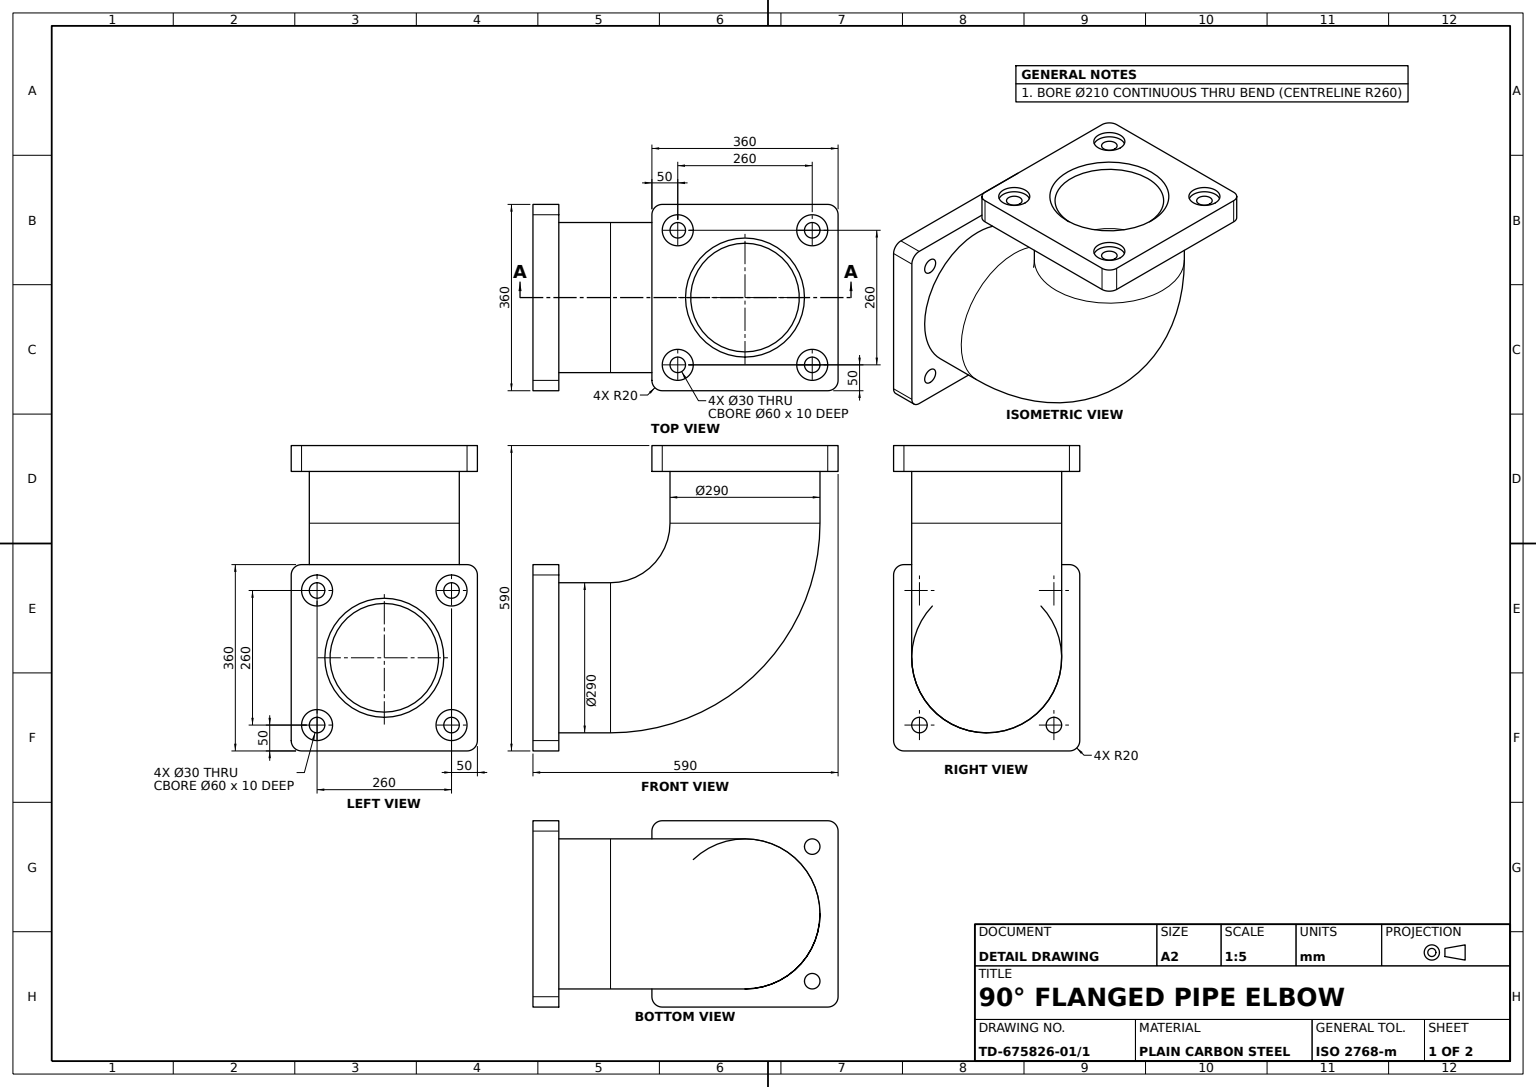
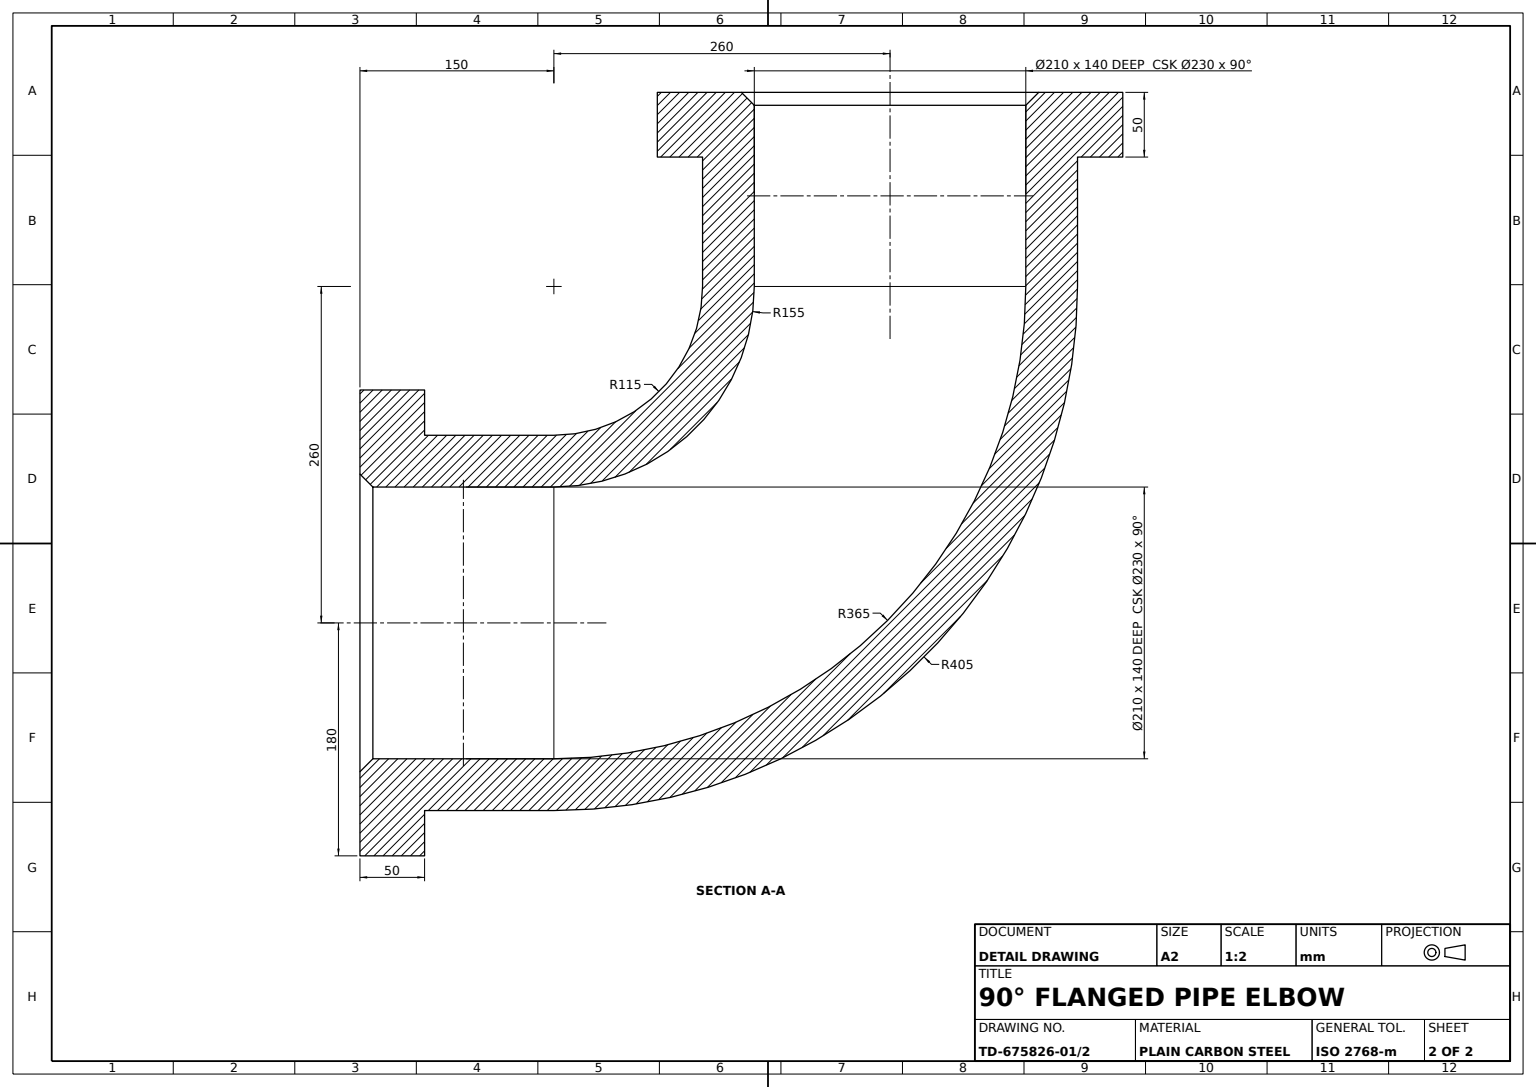
solid
v1 (0,260,-145)
v2 (-145,260,0)
e1 v1 v2 CIRCLE(AX(P(0,260,0),D(0,1,0),D(-1,0,0)),145)
v3 (0,260,145)
e2 v2 v3 CIRCLE(AX(P(0,260,0),D(0,1,0),D(-1,0,0)),145)
v4 (0,360,145)
e3 v4 v3 LINE
v5 (0,360,-145)
e4 v5 v4 CIRCLE(AX(P(0,360,0),D(0,1,0),D(-1,0,0)),145)
e5 v5 v1 LINE
face CYL(AX(P(0,410,0),D(0,-1,0),D(0,0,-1)),145) [e1 e2 -e3 -e4 e5]
v6 (-360,160,-180)
v7 (-410,160,-180)
e6 v6 v7 LINE
v8 (-360,-160,-180)
e7 v6 v8 LINE
v9 (-410,-160,-180)
e8 v8 v9 LINE
e9 v7 v9 LINE
face PLANE(AX(P(-360,160,-180),D(0,0,-1),D(0,1,0))) [-e6 e7 e8 -e9]
v10 (0,400,-105)
v11 (0,260,-105)
e10 v10 v11 LINE
v12 (0,400,105)
e11 v10 v12 CIRCLE(AX(P(0,400,0),D(0,1,0),D(0,0,1)),105)
v13 (0,260,105)
e12 v12 v13 LINE
v14 (-105,260,0)
e13 v14 v13 CIRCLE(AX(P(0,260,0),D(0,1,0),D(-1,0,0)),105)
e14 v11 v14 CIRCLE(AX(P(0,260,0),D(0,1,0),D(-1,0,0)),105)
face CYL(AX(P(0,411,0),D(0,-1,0),D(0,0,-1)),105) rev [-e10 e11 e12 -e13 -e14]
v15 (-410,115,0)
v16 (-410,-115,0)
e15 v15 v16 CIRCLE(AX(P(-410,0,0),D(1,0,0),D(0,1,0)),115)
v17 (-400,105,0)
e16 v17 v15 LINE
v18 (-400,-105,0)
e17 v18 v17 CIRCLE(AX(P(-400,0,0),D(-1,0,0),D(0,1,0)),105)
e18 v18 v16 LINE
face CONE(AX(P(-410,0,0),D(-1,0,0),D(0,-1,0)),115,0.785398163) rev [-e15 -e16 -e17 e18]
v19 (-360,-145,130)
v20 (-400,-145,130)
e19 v19 v20 LINE
v21 (-400,-115,130)
e20 v20 v21 CIRCLE(AX(P(-400,-130,130),D(-1,0,0),D(0,1,0)),15)
v22 (-360,-115,130)
e21 v22 v21 LINE
e22 v22 v19 CIRCLE(AX(P(-360,-130,130),D(1,0,0),D(0,1,0)),15)
face CYL(AX(P(-360,-130,130),D(-1,0,0),D(0,-1,0)),15) rev [e19 e20 -e21 e22]
v23 (0,410,115)
e23 v12 v23 LINE
v24 (0,410,-115)
e24 v10 v24 LINE
e25 v23 v24 CIRCLE(AX(P(0,410,0),D(0,-1,0),D(-1,0,0)),115)
face CONE(AX(P(0,400,0),D(0,1,0),D(0,0,1)),105,0.785398163) rev [-e23 -e11 e24 -e25]
v25 (180,360,-160)
v26 (160,360,-180)
e26 v25 v26 CIRCLE(AX(P(160,360,-160),D(0,1,0),D(1,0,0)),20)
v27 (160,410,-180)
e27 v26 v27 LINE
v28 (180,410,-160)
e28 v28 v27 CIRCLE(AX(P(160,410,-160),D(0,1,0),D(1,0,0)),20)
e29 v25 v28 LINE
face CYL(AX(P(160,360,-160),D(0,1,0),D(-1,0,0)),20) [e26 e27 -e28 -e29]
v29 (-145,400,130)
v30 (-115,400,130)
e30 v29 v30 CIRCLE(AX(P(-130,400,130),D(0,1,0),D(-1,0,0)),15)
v31 (-115,360,130)
e31 v31 v30 LINE
v32 (-145,360,130)
e32 v32 v31 CIRCLE(AX(P(-130,360,130),D(0,1,0),D(0,0,1)),15)
e33 v32 v29 LINE
face CYL(AX(P(-130,360,130),D(0,1,0),D(-1,0,0)),15) rev [e30 -e31 -e32 e33]
v33 (-260,-145,0)
v34 (-260,145,0)
e34 v33 v34 CIRCLE(AX(P(-260,0,0),D(1,0,0),D(0,1,0)),145)
e35 v2 v34 CIRCLE(AX(P(-260,260,0),D(0,0,-1),D(-1,0,0)),115)
v35 (145,260,0)
e36 v35 v1 CIRCLE(AX(P(0,260,0),D(0,1,0),D(-1,0,0)),145)
e37 v35 v33 CIRCLE(AX(P(-260,260,0),D(0,0,-1),D(-1,0,0)),405)
face TORUS(AX(P(-260,260,0),D(0,0,-1),D(-1,0,0)),260,145) [e34 -e35 -e1 -e36 e37]
v36 (-410,-180,-160)
e38 v9 v36 CIRCLE(AX(P(-410,-160,-160),D(-1,0,0),D(0,-1,0)),20)
v37 (-410,-180,160)
e39 v36 v37 LINE
v38 (-410,-160,180)
e40 v37 v38 CIRCLE(AX(P(-410,-160,160),D(-1,0,0),D(0,-1,0)),20)
v39 (-410,160,180)
e41 v38 v39 LINE
v40 (-410,180,160)
e42 v39 v40 CIRCLE(AX(P(-410,160,160),D(-1,0,0),D(0,1,0)),20)
v41 (-410,180,-160)
e43 v40 v41 LINE
e44 v41 v7 CIRCLE(AX(P(-410,160,-160),D(-1,0,0),D(0,-1,0)),20)
e45 v16 v15 CIRCLE(AX(P(-410,0,0),D(1,0,0),D(0,1,0)),115)
v42 (-410,100,130)
v43 (-410,160,130)
e46 v42 v43 CIRCLE(AX(P(-410,130,130),D(-1,0,0),D(0,1,0)),30)
e47 v43 v42 CIRCLE(AX(P(-410,130,130),D(-1,0,0),D(0,1,0)),30)
v44 (-410,-160,-130)
v45 (-410,-100,-130)
e48 v44 v45 CIRCLE(AX(P(-410,-130,-130),D(-1,0,0),D(0,-1,0)),30)
e49 v45 v44 CIRCLE(AX(P(-410,-130,-130),D(-1,0,0),D(0,-1,0)),30)
v46 (-410,-160,130)
v47 (-410,-100,130)
e50 v46 v47 CIRCLE(AX(P(-410,-130,130),D(-1,0,0),D(0,1,0)),30)
e51 v47 v46 CIRCLE(AX(P(-410,-130,130),D(-1,0,0),D(0,1,0)),30)
v48 (-410,100,-130)
v49 (-410,160,-130)
e52 v48 v49 CIRCLE(AX(P(-410,130,-130),D(-1,0,0),D(0,-1,0)),30)
e53 v49 v48 CIRCLE(AX(P(-410,130,-130),D(-1,0,0),D(0,-1,0)),30)
face PLANE(AX(P(-410,0,0),D(1,0,0),D(0,1,0))) rev [e9 e38 e39 e40 e41 e42 e43 e44] [e15 e45] [-e46 -e47] [-e48 -e49] [-e50 -e51] [-e52 -e53]
v50 (-400,160,130)
v51 (-400,100,130)
e54 v50 v51 CIRCLE(AX(P(-400,130,130),D(-1,0,0),D(0,1,0)),30)
e55 v51 v50 CIRCLE(AX(P(-400,130,130),D(-1,0,0),D(0,1,0)),30)
v52 (-400,145,130)
v53 (-400,115,130)
e56 v52 v53 CIRCLE(AX(P(-400,130,130),D(-1,0,0),D(0,1,0)),15)
e57 v53 v52 CIRCLE(AX(P(-400,130,130),D(-1,0,0),D(0,1,0)),15)
face PLANE(AX(P(-400,130,130),D(1,0,0),D(0,1,0))) rev [e54 e55] [-e56 -e57]
v54 (-115,360,-130)
v55 (-115,400,-130)
e58 v54 v55 LINE
v56 (-145,400,-130)
e59 v55 v56 CIRCLE(AX(P(-130,400,-130),D(0,1,0),D(-1,0,0)),15)
v57 (-145,360,-130)
e60 v57 v56 LINE
e61 v54 v57 CIRCLE(AX(P(-130,360,-130),D(0,1,0),D(0,0,1)),15)
face CYL(AX(P(-130,360,-130),D(0,1,0),D(-1,0,0)),15) rev [e58 e59 -e60 -e61]
e62 v34 v33 CIRCLE(AX(P(-260,0,0),D(1,0,0),D(0,1,0)),145)
e63 v3 v35 CIRCLE(AX(P(0,260,0),D(0,1,0),D(-1,0,0)),145)
face TORUS(AX(P(-260,260,0),D(0,0,-1),D(-1,0,0)),260,145) [e35 e62 -e37 -e63 -e2]
e64 v31 v32 CIRCLE(AX(P(-130,360,130),D(0,1,0),D(0,0,1)),15)
v58 (145,360,130)
v59 (115,360,130)
e65 v58 v59 CIRCLE(AX(P(130,360,130),D(0,-1,0),D(0,0,1)),15)
e66 v59 v58 CIRCLE(AX(P(130,360,130),D(0,-1,0),D(0,0,1)),15)
e67 v57 v54 CIRCLE(AX(P(-130,360,-130),D(0,1,0),D(0,0,1)),15)
v60 (115,360,-130)
v61 (145,360,-130)
e68 v60 v61 CIRCLE(AX(P(130,360,-130),D(0,-1,0),D(0,0,1)),15)
e69 v61 v60 CIRCLE(AX(P(130,360,-130),D(0,-1,0),D(0,0,1)),15)
v62 (-160,360,-180)
e70 v26 v62 LINE
v63 (180,360,160)
e71 v63 v25 LINE
v64 (160,360,180)
e72 v64 v63 CIRCLE(AX(P(160,360,160),D(0,1,0),D(-1,0,0)),20)
v65 (-160,360,180)
e73 v65 v64 LINE
v66 (-180,360,160)
e74 v66 v65 CIRCLE(AX(P(-160,360,160),D(0,1,0),D(-1,0,0)),20)
v67 (-180,360,-160)
e75 v67 v66 LINE
e76 v62 v67 CIRCLE(AX(P(-160,360,-160),D(0,1,0),D(-1,0,0)),20)
e77 v4 v5 CIRCLE(AX(P(0,360,0),D(0,1,0),D(-1,0,0)),145)
face PLANE(AX(P(-160,360,160),D(0,1,0),D(-1,0,0))) rev [e64 e32] [-e65 -e66] [e61 e67] [-e68 -e69] [-e70 -e26 -e71 -e72 -e73 -e74 -e75 -e76] [e77 e4]
v68 (-260,-105,0)
v69 (-260,105,0)
e78 v68 v69 CIRCLE(AX(P(-260,0,0),D(1,0,0),D(0,1,0)),105)
v70 (105,260,0)
e79 v70 v68 CIRCLE(AX(P(-260,260,0),D(0,0,-1),D(-1,0,0)),365)
e80 v70 v11 CIRCLE(AX(P(0,260,0),D(0,1,0),D(-1,0,0)),105)
e81 v14 v69 CIRCLE(AX(P(-260,260,0),D(0,0,-1),D(-1,0,0)),155)
face TORUS(AX(P(-260,260,0),D(0,0,-1),D(-1,0,0)),260,105) rev [-e78 -e79 e80 e14 e81]
v71 (-160,400,-130)
v72 (-160,410,-130)
e82 v71 v72 LINE
v73 (-100,410,-130)
e83 v72 v73 CIRCLE(AX(P(-130,410,-130),D(0,1,0),D(-1,0,0)),30)
v74 (-100,400,-130)
e84 v74 v73 LINE
e85 v71 v74 CIRCLE(AX(P(-130,400,-130),D(0,1,0),D(-1,0,0)),30)
face CYL(AX(P(-130,400,-130),D(0,1,0),D(-1,0,0)),30) rev [e82 e83 -e84 -e85]
e86 v21 v20 CIRCLE(AX(P(-400,-130,130),D(-1,0,0),D(0,1,0)),15)
v75 (-400,-100,130)
v76 (-400,-160,130)
e87 v75 v76 CIRCLE(AX(P(-400,-130,130),D(-1,0,0),D(0,1,0)),30)
e88 v76 v75 CIRCLE(AX(P(-400,-130,130),D(-1,0,0),D(0,1,0)),30)
face PLANE(AX(P(-400,-130,130),D(1,0,0),D(0,1,0))) rev [-e20 -e86] [e87 e88]
e89 v30 v29 CIRCLE(AX(P(-130,400,130),D(0,1,0),D(-1,0,0)),15)
face CYL(AX(P(-130,360,130),D(0,1,0),D(-1,0,0)),15) rev [e89 -e33 -e64 e31]
v77 (-360,115,130)
v78 (-360,145,130)
e90 v77 v78 CIRCLE(AX(P(-360,130,130),D(1,0,0),D(0,-1,0)),15)
e91 v78 v52 LINE
e92 v77 v53 LINE
face CYL(AX(P(-360,130,130),D(-1,0,0),D(0,-1,0)),15) rev [e90 e91 e56 -e92]
e93 v78 v77 CIRCLE(AX(P(-360,130,130),D(1,0,0),D(0,-1,0)),15)
face CYL(AX(P(-360,130,130),D(-1,0,0),D(0,-1,0)),15) rev [e93 e92 e57 -e91]
e94 v50 v43 LINE
e95 v51 v42 LINE
face CYL(AX(P(-400,130,130),D(-1,0,0),D(0,-1,0)),30) rev [-e94 -e55 e95 e46]
v79 (115,400,-130)
v80 (145,400,-130)
e96 v79 v80 CIRCLE(AX(P(130,400,-130),D(0,1,0),D(1,0,0)),15)
e97 v61 v80 LINE
e98 v60 v79 LINE
face CYL(AX(P(130,360,-130),D(0,1,0),D(-1,0,0)),15) rev [e96 -e97 e69 e98]
v81 (-400,100,-130)
v82 (-400,160,-130)
e99 v81 v82 CIRCLE(AX(P(-400,130,-130),D(-1,0,0),D(0,-1,0)),30)
e100 v81 v48 LINE
e101 v82 v49 LINE
face CYL(AX(P(-400,130,-130),D(-1,0,0),D(0,-1,0)),30) rev [-e99 e100 e52 -e101]
e102 v56 v55 CIRCLE(AX(P(-130,400,-130),D(0,1,0),D(-1,0,0)),15)
face CYL(AX(P(-130,360,-130),D(0,1,0),D(-1,0,0)),15) rev [e102 -e58 -e67 e60]
e103 v74 v71 CIRCLE(AX(P(-130,400,-130),D(0,1,0),D(-1,0,0)),30)
face PLANE(AX(P(-130,400,-130),D(0,1,0),D(-1,0,0))) [e103 e85] [-e102 -e59]
e104 v12 v10 CIRCLE(AX(P(0,400,0),D(0,1,0),D(0,0,1)),105)
e105 v13 v70 CIRCLE(AX(P(0,260,0),D(0,1,0),D(-1,0,0)),105)
face CYL(AX(P(0,411,0),D(0,-1,0),D(0,0,-1)),105) rev [e104 e10 -e80 -e105 -e12]
e106 v73 v72 CIRCLE(AX(P(-130,410,-130),D(0,1,0),D(-1,0,0)),30)
face CYL(AX(P(-130,400,-130),D(0,1,0),D(-1,0,0)),30) rev [e84 e106 -e82 -e103]
v83 (-360,-180,160)
e107 v83 v37 LINE
v84 (-360,-180,-160)
e108 v84 v36 LINE
e109 v84 v83 LINE
face PLANE(AX(P(-360,-180,-160),D(0,-1,0),D(1,0,0))) [e107 -e39 -e108 e109]
e110 v80 v79 CIRCLE(AX(P(130,400,-130),D(0,1,0),D(1,0,0)),15)
face CYL(AX(P(130,360,-130),D(0,1,0),D(-1,0,0)),15) rev [e110 -e98 e68 e97]
v85 (-360,180,-160)
e111 v85 v41 LINE
v86 (-360,180,160)
e112 v86 v40 LINE
e113 v86 v85 LINE
face PLANE(AX(P(-360,180,-160),D(0,1,0),D(-1,0,0))) [e111 -e43 -e112 e113]
e114 v17 v18 CIRCLE(AX(P(-400,0,0),D(-1,0,0),D(0,1,0)),105)
e115 v68 v18 LINE
e116 v69 v17 LINE
face CYL(AX(P(-260,0,0),D(-1,0,0),D(0,-1,0)),105) rev [e114 -e115 e78 e116]
v87 (-400,115,-130)
v88 (-400,145,-130)
e117 v87 v88 CIRCLE(AX(P(-400,130,-130),D(-1,0,0),D(0,-1,0)),15)
v89 (-360,145,-130)
e118 v89 v88 LINE
v90 (-360,115,-130)
e119 v90 v89 CIRCLE(AX(P(-360,130,-130),D(-1,0,0),D(0,-1,0)),15)
e120 v90 v87 LINE
face CYL(AX(P(-360,130,-130),D(-1,0,0),D(0,-1,0)),15) rev [e117 -e118 -e119 e120]
v91 (160,400,130)
v92 (100,400,130)
e121 v91 v92 CIRCLE(AX(P(130,400,130),D(0,1,0),D(1,0,0)),30)
e122 v92 v91 CIRCLE(AX(P(130,400,130),D(0,1,0),D(1,0,0)),30)
v93 (145,400,130)
v94 (115,400,130)
e123 v93 v94 CIRCLE(AX(P(130,400,130),D(0,1,0),D(1,0,0)),15)
e124 v94 v93 CIRCLE(AX(P(130,400,130),D(0,1,0),D(1,0,0)),15)
face PLANE(AX(P(130,400,130),D(0,-1,0),D(1,0,0))) rev [e121 e122] [-e123 -e124]
v95 (160,400,-130)
v96 (100,400,-130)
e125 v95 v96 CIRCLE(AX(P(130,400,-130),D(0,1,0),D(1,0,0)),30)
e126 v96 v95 CIRCLE(AX(P(130,400,-130),D(0,1,0),D(1,0,0)),30)
face PLANE(AX(P(130,400,-130),D(0,-1,0),D(1,0,0))) rev [-e96 -e110] [e125 e126]
v97 (-360,-145,0)
e127 v33 v97 LINE
v98 (-360,145,0)
e128 v34 v98 LINE
e129 v97 v98 CIRCLE(AX(P(-360,0,0),D(-1,0,0),D(0,-1,0)),145)
face CYL(AX(P(-260,0,0),D(-1,0,0),D(0,-1,0)),145) [-e127 -e62 e128 -e129]
v99 (160,410,130)
e130 v91 v99 LINE
v100 (100,410,130)
e131 v99 v100 CIRCLE(AX(P(130,410,130),D(0,1,0),D(1,0,0)),30)
e132 v92 v100 LINE
face CYL(AX(P(130,400,130),D(0,1,0),D(-1,0,0)),30) rev [-e121 e130 e131 -e132]
v101 (160,410,-130)
v102 (100,410,-130)
e133 v101 v102 CIRCLE(AX(P(130,410,-130),D(0,1,0),D(1,0,0)),30)
e134 v96 v102 LINE
e135 v95 v101 LINE
face CYL(AX(P(130,400,-130),D(0,1,0),D(-1,0,0)),30) rev [e133 -e134 -e125 e135]
e136 v76 v46 LINE
e137 v75 v47 LINE
face CYL(AX(P(-400,-130,130),D(-1,0,0),D(0,-1,0)),30) rev [-e88 e136 e50 -e137]
e138 v69 v68 CIRCLE(AX(P(-260,0,0),D(1,0,0),D(0,1,0)),105)
face CYL(AX(P(-260,0,0),D(-1,0,0),D(0,-1,0)),105) rev [e115 e17 -e116 e138]
v103 (-400,-100,-130)
e139 v103 v45 LINE
v104 (-400,-160,-130)
e140 v104 v103 CIRCLE(AX(P(-400,-130,-130),D(-1,0,0),D(0,-1,0)),30)
e141 v104 v44 LINE
face CYL(AX(P(-400,-130,-130),D(-1,0,0),D(0,-1,0)),30) rev [e48 -e139 -e140 e141]
v105 (-180,410,160)
v106 (-160,410,180)
e142 v105 v106 CIRCLE(AX(P(-160,410,160),D(0,1,0),D(-1,0,0)),20)
e143 v66 v105 LINE
e144 v65 v106 LINE
face CYL(AX(P(-160,360,160),D(0,1,0),D(-1,0,0)),20) [-e142 -e143 e74 e144]
e145 v102 v101 CIRCLE(AX(P(130,410,-130),D(0,1,0),D(1,0,0)),30)
face CYL(AX(P(130,400,-130),D(0,1,0),D(-1,0,0)),30) rev [e145 -e135 -e126 e134]
v107 (-160,400,130)
v108 (-160,410,130)
e146 v107 v108 LINE
v109 (-100,400,130)
e147 v109 v107 CIRCLE(AX(P(-130,400,130),D(0,1,0),D(-1,0,0)),30)
v110 (-100,410,130)
e148 v109 v110 LINE
e149 v110 v108 CIRCLE(AX(P(-130,410,130),D(0,1,0),D(-1,0,0)),30)
face CYL(AX(P(-130,400,130),D(0,1,0),D(-1,0,0)),30) rev [-e146 -e147 e148 e149]
e150 v19 v22 CIRCLE(AX(P(-360,-130,130),D(1,0,0),D(0,1,0)),15)
face CYL(AX(P(-360,-130,130),D(-1,0,0),D(0,-1,0)),15) rev [e86 -e19 e150 e21]
e151 v59 v94 LINE
e152 v58 v93 LINE
face CYL(AX(P(130,360,130),D(0,1,0),D(-1,0,0)),15) rev [e123 -e151 e66 e152]
face CYL(AX(P(-400,130,130),D(-1,0,0),D(0,-1,0)),30) rev [e47 -e95 -e54 e94]
v111 (180,410,160)
e153 v111 v28 LINE
e154 v63 v111 LINE
face PLANE(AX(P(180,360,-160),D(1,0,0),D(0,0,-1))) [-e153 -e154 e71 e29]
face CYL(AX(P(0,410,0),D(0,-1,0),D(0,0,-1)),145) [e63 e36 -e5 -e77 e3]
e155 v88 v87 CIRCLE(AX(P(-400,130,-130),D(-1,0,0),D(0,-1,0)),15)
e156 v89 v90 CIRCLE(AX(P(-360,130,-130),D(-1,0,0),D(0,-1,0)),15)
face CYL(AX(P(-360,130,-130),D(-1,0,0),D(0,-1,0)),15) rev [e155 -e120 -e156 e118]
e157 v103 v104 CIRCLE(AX(P(-400,-130,-130),D(-1,0,0),D(0,-1,0)),30)
face CYL(AX(P(-400,-130,-130),D(-1,0,0),D(0,-1,0)),30) rev [-e141 -e157 e139 e49]
e158 v82 v81 CIRCLE(AX(P(-400,130,-130),D(-1,0,0),D(0,-1,0)),30)
face PLANE(AX(P(-400,130,-130),D(-1,0,0),D(0,-1,0))) [e158 e99] [-e155 -e117]
face CYL(AX(P(-400,130,-130),D(-1,0,0),D(0,-1,0)),30) rev [e101 e53 -e100 -e158]
v112 (-360,-115,-130)
v113 (-400,-115,-130)
e159 v112 v113 LINE
v114 (-360,-145,-130)
e160 v114 v112 CIRCLE(AX(P(-360,-130,-130),D(-1,0,0),D(0,-1,0)),15)
v115 (-400,-145,-130)
e161 v114 v115 LINE
e162 v115 v113 CIRCLE(AX(P(-400,-130,-130),D(-1,0,0),D(0,-1,0)),15)
face CYL(AX(P(-360,-130,-130),D(-1,0,0),D(0,-1,0)),15) rev [-e159 -e160 e161 e162]
e163 v107 v109 CIRCLE(AX(P(-130,400,130),D(0,1,0),D(-1,0,0)),30)
face PLANE(AX(P(-130,400,130),D(0,1,0),D(-1,0,0))) [-e89 -e30] [e147 e163]
e164 v108 v110 CIRCLE(AX(P(-130,410,130),D(0,1,0),D(-1,0,0)),30)
face CYL(AX(P(-130,400,130),D(0,1,0),D(-1,0,0)),30) rev [-e148 -e163 e146 e164]
e165 v24 v23 CIRCLE(AX(P(0,410,0),D(0,-1,0),D(-1,0,0)),115)
face CONE(AX(P(0,400,0),D(0,1,0),D(0,0,1)),105,0.785398163) rev [-e104 e23 -e165 -e24]
face TORUS(AX(P(-260,260,0),D(0,0,-1),D(-1,0,0)),260,105) rev [e105 e79 -e138 -e81 e13]
e166 v100 v99 CIRCLE(AX(P(130,410,130),D(0,1,0),D(1,0,0)),30)
v116 (160,410,180)
e167 v116 v111 CIRCLE(AX(P(160,410,160),D(0,1,0),D(-1,0,0)),20)
v117 (-160,410,-180)
e168 v27 v117 LINE
v118 (-180,410,-160)
e169 v117 v118 CIRCLE(AX(P(-160,410,-160),D(0,1,0),D(-1,0,0)),20)
e170 v118 v105 LINE
e171 v106 v116 LINE
face PLANE(AX(P(0,410,0),D(0,1,0),D(-1,0,0))) [-e131 -e166] [e25 e165] [-e149 -e164] [-e133 -e145] [-e83 -e106] [e167 e153 e28 e168 e169 e170 e142 e171]
face CYL(AX(P(130,400,130),D(0,1,0),D(-1,0,0)),30) rev [-e122 e132 e166 -e130]
e172 v85 v6 CIRCLE(AX(P(-360,160,-160),D(-1,0,0),D(0,-1,0)),20)
face CYL(AX(P(-360,160,-160),D(-1,0,0),D(0,-1,0)),20) [-e111 e172 e6 -e44]
face CYL(AX(P(130,360,130),D(0,1,0),D(-1,0,0)),15) rev [e65 e151 e124 -e152]
e173 v98 v97 CIRCLE(AX(P(-360,0,0),D(-1,0,0),D(0,-1,0)),145)
v119 (-360,160,180)
e174 v119 v86 CIRCLE(AX(P(-360,160,160),D(-1,0,0),D(0,1,0)),20)
v120 (-360,-160,180)
e175 v120 v119 LINE
e176 v83 v120 CIRCLE(AX(P(-360,-160,160),D(-1,0,0),D(0,-1,0)),20)
e177 v8 v84 CIRCLE(AX(P(-360,-160,-160),D(-1,0,0),D(0,-1,0)),20)
e178 v112 v114 CIRCLE(AX(P(-360,-130,-130),D(-1,0,0),D(0,-1,0)),15)
face PLANE(AX(P(-360,-160,-160),D(-1,0,0),D(0,-1,0))) rev [e156 e119] [-e90 -e93] [e129 e173] [-e150 -e22] [-e172 -e113 -e174 -e175 -e176 -e109 -e177 -e7] [e160 e178]
e179 v113 v115 CIRCLE(AX(P(-400,-130,-130),D(-1,0,0),D(0,-1,0)),15)
face PLANE(AX(P(-400,-130,-130),D(-1,0,0),D(0,-1,0))) [e140 e157] [-e179 -e162]
e180 v62 v117 LINE
e181 v67 v118 LINE
face CYL(AX(P(-160,360,-160),D(0,1,0),D(-1,0,0)),20) [-e180 e76 e181 -e169]
face CONE(AX(P(-410,0,0),D(-1,0,0),D(0,-1,0)),115,0.785398163) rev [e16 -e45 -e18 -e114]
e182 v120 v38 LINE
e183 v119 v39 LINE
face PLANE(AX(P(-360,160,180),D(0,0,1),D(0,-1,0))) [-e182 e175 e183 -e41]
face CYL(AX(P(-360,-160,160),D(-1,0,0),D(0,-1,0)),20) [-e107 e176 e182 -e40]
face PLANE(AX(P(-160,360,-180),D(0,0,-1),D(-1,0,0))) [-e27 e70 e180 -e168]
face CYL(AX(P(-360,160,160),D(-1,0,0),D(0,-1,0)),20) [-e183 e174 e112 -e42]
face PLANE(AX(P(-180,360,-160),D(-1,0,0),D(0,0,1))) [-e170 -e181 e75 e143]
e184 v64 v116 LINE
face PLANE(AX(P(-160,360,180),D(0,0,1),D(1,0,0))) [e184 -e171 -e144 e73]
face CYL(AX(P(-260,0,0),D(-1,0,0),D(0,-1,0)),145) [-e173 -e128 -e34 e127]
face CYL(AX(P(-400,-130,130),D(-1,0,0),D(0,-1,0)),30) rev [e51 -e136 -e87 e137]
face CYL(AX(P(-360,-130,-130),D(-1,0,0),D(0,-1,0)),15) rev [-e178 e159 e179 -e161]
face CYL(AX(P(-360,-160,-160),D(-1,0,0),D(0,-1,0)),20) [e177 e108 -e38 -e8]
face CYL(AX(P(160,360,160),D(0,1,0),D(-1,0,0)),20) [-e167 -e184 e72 e154]
